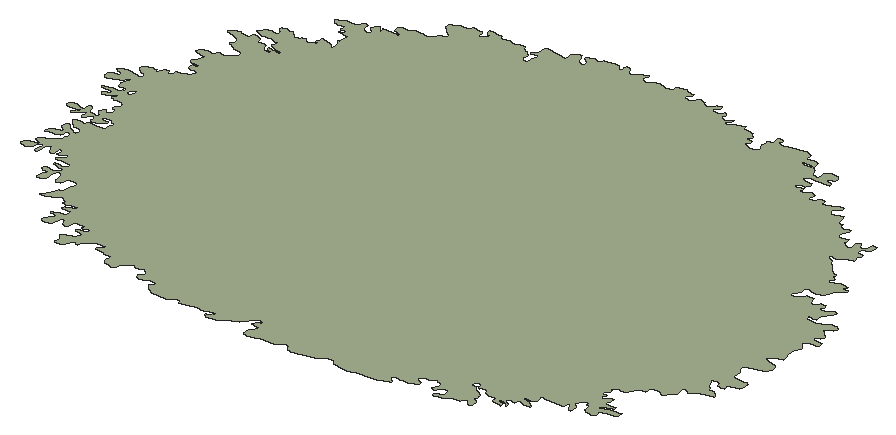
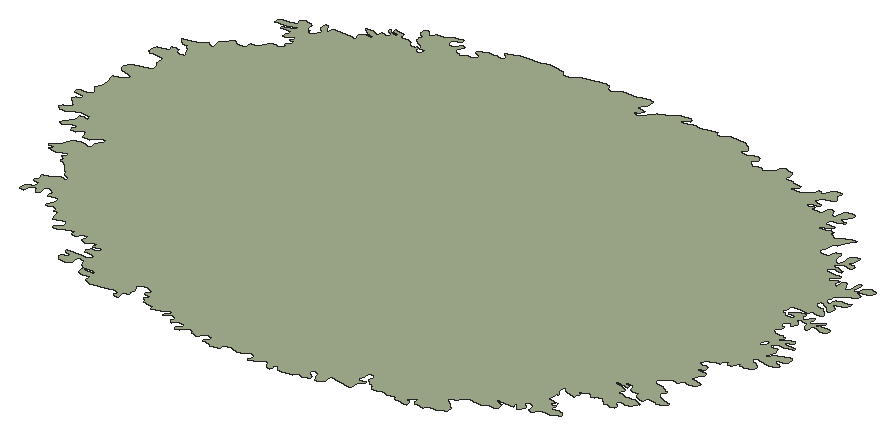
# SketchUp Ruby script. Lengths in inches.
U = 1.inch
M = Sketchup.active_model
def pt(a) = Geom::Point3d.new(a.map { |v| v * U })
def face(e, loops, mat)
  f = e.add_face(loops[0].map { |a| pt(a) })
  loops[1..].each { |l| e.add_face(l.map { |a| pt(a) }).erase! }
  f.material = f.back_material = mat if mat
  f
end
# faces: each face lists its corners as indices into pts; further lists are holes
def faces(e, pts, list, mat = nil) = list.each { |f| face(e, (f[0].is_a?(Array) ? f : [f]).map { |l| l.map { |i| pts[i] } }, mat) }
# xy, xz, yz: faces in a plane at the given z, y or x. An outline is a flat list of corners, or four numbers for a rectangle; further outlines are holes
def ring(l) = l.size == 4 ? [[l[0], l[1]], [l[2], l[1]], [l[2], l[3]], [l[0], l[3]]] : l.each_slice(2).to_a
def flat(e, list, mat, &to3) = list.each { |f| face(e, (f[0].is_a?(Array) ? f : [f]).map { |l| ring(l).map { |u, v| to3.(u, v) } }, mat) }
def xy(e, z, list, mat = nil) = flat(e, list, mat) { |x, y| [x, y, z] }
def xz(e, y, list, mat = nil) = flat(e, list, mat) { |x, z| [x, y, z] }
def yz(e, x, list, mat = nil) = flat(e, list, mat) { |y, z| [x, y, z] }
def lines(e, pts, list) = list.each { |a, b| e.add_line(pt(pts[a]), pt(pts[b])) }
# prism: a flat outline (further loops are holes) pulled along v
def prism(e, loops, v, mat = nil)
  f = face(e, loops, mat); d = Geom::Vector3d.new(v.map { |x| x * U })
  f.pushpull(f.normal.samedirection?(d) ? d.length : -d.length)
end
def box(e, o, s, mat = nil) = prism(e, [[o, [o[0] + s[0], o[1], o[2]], [o[0] + s[0], o[1] + s[1], o[2]], [o[0], o[1] + s[1], o[2]]]], [0, 0, s[2]], mat)
def at(x, y, z, deg = 0) = Geom::Transformation.translation(pt([x, y, z])) * Geom::Transformation.rotation(ORIGIN, Z_AXIS, deg.degrees)
def axes(o, x, y, z) = Geom::Transformation.new([*x, 0, *y, 0, *z, 0, *pt(o).to_a, 1])
def part(name) = M.definitions.add(name)
# library, detail: a bought-in or finely detailed component or shape, given as its bounding box
def library(name, o, s) = part(name).tap { |d| box(d.entities, o, s) }
def detail(e, o, s) = box(e.add_group.entities, o, s)
def put(e, d, t, mat = nil) = e.add_instance(d, t).tap { |i| i.material = mat if mat }
def group(e, t, mat = nil) = e.add_group.tap { |g| g.transformation = t; g.material = mat if mat }.entities
root = M.entities
M.materials.add("Boxwoodplan").color = [166, 177, 144]
xy(root,9.058,[[[143.917,67.129,143.806,67.133,143.711,67.159,143.655,67.215,143.653,67.317,143.679,67.382,143.743,67.445,143.792,67.509,143.85,67.606,143.664,67.635,143.574,67.644,143.594,67.732,143.68,67.79,143.711,67.8,143.706,67.846,143.617,67.877,143.501,67.837,143.404,67.706,143.261,67.551,143.1,67.464,142.995,67.441,142.934,67.416,142.918,67.373,142.774,67.281,142.58,67.251,142.491,67.26,142.411,67.306,142.411,67.328,142.456,67.359,142.547,67.437,142.615,67.483,142.526,67.498,142.413,67.48,142.293,67.436,142.197,67.445,142.1,67.454,142.003,67.447,141.876,67.403,141.676,67.356,141.587,67.349,141.549,67.443,141.541,67.465,141.474,67.473,141.385,67.454,141.216,67.336,141.016,67.328,140.786,67.353,140.619,67.446,140.478,67.61,140.661,67.702,140.561,67.756,140.425,67.772,140.299,67.749,140.227,67.697,140.146,67.672,140.03,67.738,139.988,67.806,140.076,67.847,140.102,67.907,140.107,67.957,140.066,68.009,139.994,68.085,139.908,68.117,139.821,68.064,139.755,68.038,139.699,68.08,139.682,68.103,139.658,68.121,139.629,68.111,139.549,68.058,139.478,68.01,139.402,67.923,139.39,67.79,139.319,67.749,139.269,67.723,139.209,67.725,139.11,67.746,139.023,67.793,138.979,67.861,138.971,67.951,138.98,68.018,138.993,68.04,138.974,68.08,138.76,68.1,138.828,68.135,138.802,68.136,138.709,68.13,138.539,68.146,138.462,68.173,138.445,68.206,138.46,68.224,138.585,68.314,138.583,68.371,138.498,68.393,138.339,68.39,138.208,68.319,138.111,68.233,138.036,68.199,137.989,68.172,137.988,68.154,138.024,68.101,138.008,68.046,137.938,68.081,137.874,68.121,137.813,68.072,137.791,68.017,137.759,67.904,137.712,67.855,137.639,67.822,137.548,67.816,137.478,67.841,137.459,67.874,137.466,67.892,137.487,67.932,137.509,67.991,137.478,68.048,137.377,68.149,137.491,68.229,137.552,68.269,137.632,68.285,137.699,68.315,137.754,68.37,137.839,68.476,137.767,68.503,137.6875,68.511,137.555,68.53,137.517,68.565,137.524,68.584,137.599,68.62,137.761,68.657,137.803,68.709,137.798,68.748,137.772,68.764,137.622,68.711,137.576,68.732,137.577,68.752,137.6,68.814,137.439,68.825,137.358,68.833,137.304,68.826,137.297,68.806,137.281,68.71,137.266,68.642,137.224,68.591,137.177,68.578,137.158,68.594,137.099,68.639,137.054,68.757,137.015,68.783,136.988,68.784,136.934,68.777,136.927,68.757,136.925,68.641,136.871,68.523,136.81,68.449,136.73,68.419,136.651,68.422,136.605,68.448,136.572,68.506,136.572,68.564,136.626,68.677,136.74,68.784,136.76,68.803,136.747,68.823,136.72,68.829,136.64,68.847,136.559,68.86,136.532,68.875,136.539,68.895,136.559,68.914,136.708,68.982,136.87,69.005,136.912,69.108,136.885,69.169,136.838,69.191,136.811,69.187,136.648,69.168,136.607,69.2,136.614,69.22,136.641,69.279,136.799,69.334,136.971,69.403,137.019,69.442,137.006,69.463,136.909,69.436,136.738,69.417,136.594,69.372,136.505,69.386,136.478,69.392,136.484,69.412,136.505,69.426,136.56,69.47,136.532,69.507,136.505,69.503,136.422,69.511,136.367,69.56,136.353,69.601,136.326,69.597,136.243,69.575,136.086,69.489,135.937,69.413,135.863,69.38,135.808,69.392,135.821,69.412,135.84,69.452,135.867,69.469,135.891,69.55,135.941,69.65,135.973,69.759,136.024,69.812,136.097,69.852,136.141,69.972,136.163,70.112,136.183,70.227,136.179,70.285,136.134,70.321,136.053,70.335,135.967,70.335,135.893,70.31,135.883,70.245,135.884,70.184,135.851,70.124,135.763,70.087,135.706,70.096,135.668,70.155,135.657,70.216,135.631,70.337,135.626,70.4,135.585,70.453,135.558,70.475,135.52,70.491,135.461,70.479,135.427,70.46,135.425,70.428,135.417,70.366,135.42,70.229,135.445,70.167,135.437,70.103,135.386,70.038,135.338,70.01,135.3,69.998,135.262,70.003,135.22,70.011,135.202,70.039,135.198,70.166,135.219,70.223,135.264,70.276,135.28,70.306,135.272,70.334,135.215,70.34,135.133,70.346,135.096,70.362,135.073,70.39,135.07,70.453,135.085,70.483,135.12,70.499,135.292,70.472,135.371,70.497,135.42,70.526,135.481,70.573,135.494,70.636,135.471,70.662,135.427,70.664,135.35,70.67,135.258,70.681,135.157,70.717,135.138,70.746,135.144,70.76,135.163,70.763,135.223,70.775,135.398,70.761,135.488,70.787,135.5,70.844,135.474,70.907,135.402,70.946,135.323,70.953,135.21,70.946,135.11,70.921,135.027,70.939,135.023,70.968,135.043,70.997,135.09,71.054,135.156,71.11,135.209,71.19,135.201,71.224,135.156,71.241,135.091,71.24,134.973,71.14,134.933,71.141,134.899,71.161,134.921,71.22,134.937,71.287,134.894,71.35,134.854,71.366,134.834,71.367,134.828,71.352,134.832,71.306,134.829,71.164,134.788,71.102,134.749,71.108,134.714,71.131,134.616,71.262,134.592,71.327,134.567,71.355,134.552,71.344,134.496,71.293,134.461,71.234,134.481,71.103,134.486,71.037,134.466,70.971,134.416,70.962,134.382,70.978,134.372,71.023,134.392,71.155,134.401,71.233,134.401,71.27,134.386,71.282,134.371,71.272,134.292,71.237,134.252,71.183,134.243,71.12,134.204,71.077,134.067,70.987,134.027,70.977,133.983,70.986,133.903,71.026,133.883,71.056,133.887,71.089,133.92,71.151,134.017,71.237,134.107,71.263,134.197,71.263,134.292,71.267,134.231,71.318,134.08,71.404,134.063,71.466,134.116,71.503,134.208,71.573,134.327,71.635,134.445,71.709,134.481,71.723,134.507,71.746,134.533,71.789,134.536,71.882,134.569,72.003,134.57,72.065,134.549,72.086,134.527,72.095,134.464,72.109,134.431,72.104,134.427,72.088,134.439,71.996,134.397,71.934,134.349,71.899,134.272,71.871,134.201,71.858,134.04,71.833,134.005,71.839,133.992,71.853,133.992,71.86,134.001,71.901,134.018,71.947,134.06,71.995,134.129,72.042,134.188,72.063,134.246,72.065,134.285,72.068,134.305,72.075,134.328,72.096,134.323,72.121,134.269,72.151,134.201,72.207,134.169,72.264,134.165,72.331,134.178,72.382,134.23,72.426,134.256,72.432,134.267,72.425,134.287,72.411,134.33,72.35,134.379,72.304,134.507,72.226,134.581,72.192,134.616,72.177,134.636,72.184,134.66,72.206,134.667,72.222,134.678,72.263,134.663,72.32,134.62,72.366,134.588,72.389,134.554,72.401,134.494,72.401,134.42,72.404,134.377,72.446,134.291,72.519,134.232,72.569,134.193,72.617,134.194,72.646,134.218,72.671,134.274,72.698,134.309,72.703,134.35,72.7,134.41,72.679,134.472,72.677,134.508,72.684,134.542,72.726,134.591,72.757,134.65,72.764,134.721,72.764,134.875,72.771,135.015,72.792,135.048,72.808,135.049,72.826,135.043,72.868,135.031,72.913,135.042,72.957,135.072,73.06,135.059,73.083,135.036,73.097,134.979,73.126,134.926,73.164,134.853,73.192,134.78,73.195,134.73,73.184,134.709,73.17,134.684,73.119,134.689,73.098,134.7,73.093,134.724,73.088,134.875,73.076,134.901,73.071,134.906,73.0625,134.897,73.046,134.857,73.007,134.812,72.964,134.747,72.928,134.685,72.884,134.613,72.849,134.576,72.852,134.556,72.863,134.531,72.9,134.524,72.995,134.507,73.02,134.525,73.034,134.531,73.077,134.525,73.088,134.514,73.088,134.499,73.087,134.473,73.083,134.441,73.076,134.423,73.065,134.342,72.97,134.31,72.915,134.279,72.892,134.256,72.895,134.23,72.916,134.221,72.932,134.215,72.973,134.244,73.057,134.249,73.102,134.24,73.13,134.22,73.137,134.182,73.128,134.162,73.114,134.116,73.064,133.994,72.957,133.958,72.932,133.932,72.927,133.895,72.935,133.883,72.951,133.974,73.057,134.037,73.102,134.051,73.129,134.05,73.145,134.041,73.152,134.03,73.148,134.015,73.143,133.984,73.131,133.9,73.108,133.733,73.089,133.66,73.096,133.612,73.121,133.59,73.149,133.589,73.165,133.606,73.217,133.654,73.264,133.714,73.281,133.785,73.284,133.859,73.266,133.987,73.223,134.073,73.197,134.084,73.201,134.084,73.22,134.075,73.239,134.05,73.287,134.049,73.342,134.056,73.407,134.068,73.437,134.085,73.45,134.134,73.413,134.173,73.363,134.2,73.317,134.21,73.255,134.222,73.204,134.237,73.176,134.26,73.175,134.395,73.157,134.468,73.144,134.503,73.14,134.521,73.154,134.536,73.202,134.481,73.244,134.422,73.309,134.405,73.335,134.405,73.352,134.439,73.46,134.469,73.483,134.496,73.489,134.511,73.477,134.52,73.459,134.549,73.414,134.56,73.39,134.572,73.391,134.593,73.404,134.673,73.482,134.69,73.528,134.691,73.579,134.677,73.611,134.656,73.623,134.593,73.646,134.553,73.666,134.545,73.687,134.561,73.736,134.617,73.773,134.651,73.795,134.664,73.816,134.672,73.869,134.67,73.916,134.575,73.992,134.431,74.014,134.369,74.031,134.334,74.013,134.306,74.014,134.237,74.031,134.218,74.058,134.227,74.082,134.353,74.185,134.347,74.217,134.325,74.233,134.28,74.225,134.251,74.216,134.125,74.154,134.085,74.107,134.036,74.063,133.967,74.049,133.939,74.05,133.892,74.102,133.92,74.126,133.9375,74.165,133.969,74.188,134.063,74.22,134.108,74.25,134.097,74.281,134.084,74.283,134.074,74.276,134.048,74.27,134.009,74.273,133.874,74.284,133.727,74.3125,133.703,74.327,133.709,74.347,133.734,74.375,133.947,74.435,134.01,74.434,134.071,74.419,134.131,74.391,134.158,74.393,134.164,74.403,134.213,74.48,134.237,74.495,134.243,74.515,134.243,74.583,134.232,74.593,134.219,74.591,134.161,74.591,134.104,74.585,134.057,74.568,134.033,74.576,134.012,74.596,133.987,74.63,133.967,74.718,133.978,74.806,134.008,74.848,134.014,74.88,134.027,74.923,134.064,74.944,134.06,74.99,134.038,75.026,133.949,75.003,133.931,74.969,133.932,74.95,133.935,74.886,133.855,74.839,133.714,74.745,133.558,74.7,133.474,74.725,133.432,74.778,133.423,74.904,133.551,74.99,133.634,75.003,133.677,75.027,133.701,75.061,133.7,75.081,133.614,75.112,133.541,75.138,133.479,75.194,133.514,75.249,133.59,75.278,133.686,75.312,133.751,75.311,133.93,75.267,134.022,75.246,134.107,75.25,134.158,75.269,134.164,75.289,134.148,75.355,134.087,75.407,134.042,75.415,133.93,75.485,133.883,75.527,133.869,75.564,133.862,75.617,133.862,75.644,133.875,75.659,133.917,75.695,133.968,75.709,134.082,75.741,134.113,75.751,134.153,75.75,134.203,75.746,134.216,75.733,134.231,75.703,134.245,75.689,134.255,75.689,134.283,75.692,134.299,75.704,134.32,75.754,134.348,75.787,134.364,75.81,134.367,75.835,134.383,75.86,134.403,75.872,134.451,75.884,134.49,75.877,134.511,75.833,134.515,75.781,134.532,75.755,134.553,75.754,134.595,75.796,134.62,75.838,134.634,75.942,134.65,75.968,134.682,75.975,134.714,75.974,134.733,75.963,134.754,75.94,134.786,75.94,134.839,75.961,134.883,76.007,134.897,76.032,134.886,76.046,134.946,76.043,134.975,76.046,134.991,76.066,134.996,76.114,135.03,76.155,135.064,76.2,135.01,76.243,134.943,76.272,134.906,76.271,134.873,76.261,134.831,76.249,134.789,76.255,134.767,76.271,134.746,76.295,134.723,76.397,134.736,76.423,134.741,76.439,134.751,76.443,134.856,76.463,134.902,76.472,134.92,76.483,134.91,76.486,134.824,76.514,134.758,76.526,134.73,76.519,134.695,76.52,134.659,76.52,134.623,76.532,134.585,76.582,134.567,76.611,134.567,76.642,134.582,76.663,134.611,76.678,134.642,76.697,134.65,76.725,134.68,76.782,134.707,76.836,134.713,76.89,134.706,76.917,134.666,76.928,134.588,76.954,134.415,77.001,134.379,77.018,134.362,77.042,134.398,77.097,134.442,77.131,134.488,77.159,134.543,77.178,134.595,77.1875,134.648,77.184,134.703,77.16,134.758,77.162,134.785,77.167,134.798,77.187,134.815,77.228,134.852,77.264,134.873,77.282,134.899,77.284,134.968,77.267,135.03,77.256,135.056,77.253,135.08,77.268,135.167,77.336,135.254,77.401,135.308,77.498,135.304,77.542,135.263,77.579,135.146,77.617,135.02,77.647,134.934,77.719,134.876,77.755,134.807,77.776,134.78,77.788,134.766,77.808,134.788,77.855,134.836,77.896,134.834,77.981,134.784,78.06,134.654,78.116,134.366,78.212,134.345,78.246,134.417,78.31,134.538,78.362,134.643,78.367,134.7,78.353,134.744,78.327,134.793,78.317,134.846,78.326,134.907,78.337,134.936,78.368,134.951,78.448,134.968,78.483,135.022,78.482,135.079,78.471,135.127,78.451,135.194,78.392,135.218,78.358,135.232,78.318,135.233,78.249,135.239,78.245,135.248,78.249,135.275,78.262,135.326,78.268,135.415,78.271,135.495,78.235,135.529,78.17,135.554,78.092,135.624,78.047,135.664,78.035,135.682,78.034,135.709,78.043,135.804,78.05,135.821,78.055,135.801,78.071,135.738,78.095,135.686,78.099,135.648,78.118,135.629,78.152,135.626,78.164,135.629,78.184,135.644,78.191,135.679,78.192,135.721,78.185,135.827,78.156,135.942,78.152,135.994,78.159,136.012,78.162,136.038,78.173,135.994,78.203,135.953,78.213,135.867,78.228,135.809,78.242,135.768,78.244,135.746,78.248,135.721,78.263,135.669,78.289,135.622,78.315,135.6,78.348,135.61,78.404,135.639,78.442,135.68,78.471,135.64,78.502,135.585,78.517,135.542,78.52,135.487,78.528,135.456,78.555,135.438,78.591,135.424,78.6,135.395,78.599,135.279,78.571,135.227,78.557,135.178,78.559,135.13,78.562,135.081,78.578,135.033,78.595,134.993,78.602,134.907,78.65,134.932,78.662,134.934,78.669,134.945,78.709,134.961,78.745,134.987,78.782,135.018,78.814,135.062,78.839,135.115,78.862,135.16,78.873,135.266,78.867,135.343,78.862,135.376,78.858,135.387,78.857,135.387,78.87,135.379,78.912,135.358,78.956,135.322,78.995,135.279,79.026,135.246,79.073,135.248,79.096,135.259,79.117,135.306,79.147,135.358,79.17,135.385,79.169,135.411,79.163,135.465,79.148,135.533,79.142,135.58,79.127,135.604,79.114,135.622,79.095,135.666,79.055,135.705,79.02,135.75,78.989,135.806,78.976,135.86,78.981,135.905,79.01,135.937,79.046,135.986,79.084,136.012,79.083,136.034,79.069,136.075,79.027,136.122,78.994,136.25,79.019,136.324,79.037,136.365,79.065,136.371,79.085,136.35,79.102,136.299,79.124,136.289,79.147,136.297,79.169,136.313,79.214,136.32,79.273,136.324,79.299,136.347,79.315,136.374,79.316,136.404,79.308,136.446,79.288,136.58,79.248,136.641,79.226,136.68,79.193,136.707,79.153,136.722,79.13,136.729,79.123,136.738,79.126,136.746,79.131,136.779,79.176,136.785,79.212,136.775,79.315,136.753,79.362,136.729,79.397,136.694,79.436,136.684,79.466,136.695,79.477,136.706,79.475,136.728,79.476,136.727,79.484,136.732,79.508,136.725,79.549,136.71,79.705,136.712,79.782,136.597,79.802,136.5,79.804,136.4375,79.8125,136.42,79.819,136.406,79.83,136.419,79.839,136.532,79.882,136.566,79.911,136.565,79.924,136.542,79.948,136.506,79.952,136.453,79.94,136.405,79.918,136.388,79.919,136.373,79.945,136.399,80.028,136.402,80.069,136.401,80.082,136.377,80.103,136.288,80.085,136.175,80.088,136.066,80.105,136.005,80.185,136.003,80.213,136.041,80.25,136.137,80.303,136.186,80.33,136.24,80.335,136.365,80.332,136.456,80.337,136.516,80.346,136.556,80.384,136.596,80.418,136.604,80.461,136.63,80.5,136.686,80.513,136.723,80.509,136.766,80.475,136.777,80.389,136.784,80.3,136.808,80.257,136.863,80.231,136.955,80.212,137.01,80.234,137.028,80.276,137.005,80.319,136.958,80.355,136.902,80.442,136.938,80.521,137.012,80.603,137.031,80.606,137.055,80.576,137.074,80.528,137.148,80.447,137.176,80.421,137.167,80.475,137.149,80.57,137.205,80.587,137.266,80.582,137.393,80.578,137.506,80.575,137.628,80.557,137.646,80.557,137.634,80.587,137.583,80.629,137.453,80.681,137.415,80.689,137.392,80.735,137.394,80.826,137.429,80.871,137.478,80.896,137.594,80.901,137.691,80.91,137.786,80.977,137.912,80.982,138.028,80.971,138.124,80.953,138.245,80.946,138.288,80.991,138.301,81.038,138.344,81.133,138.433,81.187,138.553,81.244,138.565,81.26,138.548,81.294,138.507,81.332,138.4,81.413,138.332,81.487,138.274,81.528,138.217,81.57,138.248,81.577,138.247,81.591,138.242,81.612,138.231,81.679,138.234,81.709,138.269,81.744,138.352,81.785,138.435,81.821,138.473,81.827,138.529,81.826,138.616,81.816,138.639,81.808,138.663,81.81,138.695,81.843,138.747,81.918,138.783,81.932,138.84,81.936,138.942,81.93,139.038,81.898,139.07,81.877,139.099,81.835,139.1,81.765,139.103,81.736,139.108,81.715,139.131,81.704,139.184,81.715,139.229,81.745,139.291,81.798,139.316,81.822,139.337,81.834,139.35,81.85,139.265,81.897,139.227,81.913,139.184,81.956,139.159,82.036,139.16,82.067,139.218,82.083,139.41,82.055,139.507,82.039,139.542,82.026,139.542,81.98,139.552,81.952,139.612,81.948,139.716,81.962,139.818,81.975,139.86,81.971,139.907,81.957,139.934,81.934,139.959,81.933,139.984,81.943,140.128,81.972,140.169,81.981,140.221,81.987,140.257,81.984,140.302,81.957,140.332,81.886,140.358,81.863,140.403,81.844,140.443,81.833,140.483,81.808,140.535,81.753,140.589,81.696,140.576,81.619,140.569,81.545,140.583,81.515,140.614,81.485,140.641,81.461,140.688,81.453,140.724,81.45,140.769,81.481,140.782,81.512,140.783,81.553,140.771,81.628,140.808,81.787,140.797,81.817,140.779,81.829,140.755,81.833,140.716,81.834,140.664,81.828,140.628,81.826,140.581,81.835,140.556,81.858,140.563,81.88,140.591,81.896,140.63,81.91,140.675,81.937,140.7,82.013,140.704,82.178,140.704,82.21,140.727,82.228,140.753,82.233,140.852,82.222,141.051,82.201,141.142,82.19,141.231,82.169,141.318,82.153,141.369,82.147,141.364,82.355,141.432,82.427,141.517,82.486,141.571,82.477,141.599,82.441,141.647,82.37,141.67,82.297,141.678,82.26,141.676,82.241,141.703,82.206,141.808,82.173,141.86,82.173,141.899,82.204,141.902,82.279,141.799,82.36,141.721,82.419,141.733,82.453,141.777,82.49,141.871,82.541,141.921,82.55,142.002,82.538,142.106,82.537,142.129,82.615,142.339,82.643,142.439,82.661,142.547,82.647,142.626,82.578,142.659,82.543,142.686,82.541,142.726,82.568,142.724,82.643,142.715,82.685,142.728,82.72,142.778,82.729,142.833,82.715,142.904,82.621,142.925,82.548,142.958,82.513,143.007,82.498,143.058,82.503,143.104,82.53,143.192,82.613,143.273,82.668,143.375,82.715,143.423,82.7,143.437,82.663,143.385,82.592,143.359,82.557,143.367,82.515,143.456,82.457,143.556,82.443,143.606,82.452,143.656,82.498,143.734,82.566,143.849,82.581,143.964,82.553,143.995,82.523,144.072,82.492,144.172,82.511,144.254,82.565,144.254,82.678,144.311,82.721,144.424,82.745,144.529,82.74,144.61,82.681,144.756,82.66,144.81,82.651,144.816,82.614,144.742,82.546,144.709,82.473,144.721,82.437,144.793,82.396,144.895,82.401,144.948,82.433,144.968,82.472,144.988,82.544,145.037,82.567,145.061,82.579,145.112,82.579,145.215,82.541,145.258,82.47,145.344,82.417,145.474,82.447,145.509,82.478,145.515,82.52,145.555,82.603,145.662,82.622,145.692,82.592,145.698,82.55,145.645,82.466,145.597,82.448,145.57,82.413,145.63,82.349,145.761,82.337,145.852,82.373,145.919,82.444,145.944,82.45,145.953,82.433,145.971,82.392,145.995,82.357,145.984,82.301,145.964,82.257,145.982,82.222,146.071,82.179,146.179,82.184,146.234,82.203,146.285,82.258,146.302,82.273,146.304,82.255,146.291,82.212,146.218,82.132,146.184,82.102,146.195,82.066,146.242,82.047,146.3,82.048,146.396,82.088,146.478,82.146,146.698,82.225,146.72,82.153,146.743,82.123,146.794,82.118,146.91,82.11,147.034,82.084,147.049,82.013,147.072,81.983,147.118,81.964,147.141,81.93,147.127,81.892,147.1,81.795,147.217,81.773,147.263,81.755,147.273,81.72,147.199,81.65,147.185,81.613,147.201,81.579,147.277,81.527,147.38,81.5,147.481,81.496,147.593,81.563,147.635,81.639,147.577,81.71,147.544,81.779,147.564,81.885,147.573,81.922,147.544,81.956,147.54,81.992,147.582,82.018,147.683,82.022,147.672,82.122,147.63,82.274,147.68,82.287,147.745,82.275,147.798,82.256,147.829,82.199,147.779,82.131,147.783,82.095,147.829,82.076,147.937,82.076,148.067,82.111,148.574,82.178,148.62,82.168,148.666,82.145,148.712,82.121,148.746,82.097,148.777,82.027,148.76,81.935,148.964,81.949,149.029,81.943,149.114,81.911,149.151,81.805,149.136,81.757,149.12,81.724,149.079,81.717,148.909,81.749,148.845,81.755,148.802,81.755,148.782,81.749,148.779,81.733,148.807,81.685,148.848,81.666,148.895,81.666,149.068,81.681,149.137,81.683,149.221,81.648,149.258,81.609,149.289,81.546,149.357,81.437,149.436,81.398,149.521,81.394,149.552,81.435,149.546,81.518,149.528,81.571,149.535,81.637,149.576,81.687,149.677,81.719,149.786,81.732,149.875,81.701,149.923,81.659,149.957,81.597,149.958,81.551,149.896,81.495,149.83,81.482,149.789,81.471,149.757,81.437,149.761,81.407,149.81,81.389,149.908,81.363,149.979,81.339,149.999,81.306,149.987,81.275,149.933,81.247,149.846,81.24,149.684,81.233,149.597,81.222,149.508,81.256,149.444,81.269,149.362,81.251,149.306,81.208,149.304,81.143,149.362,81.103,149.449,81.081,149.535,81.066,149.582,81.066,149.616,81.046,149.637,81.003,149.62,80.938,149.585,80.89,149.557,80.866,149.512,80.854,149.37,80.834,149.35,80.829,149.341,80.784,149.345,80.751,149.39,80.732,149.457,80.731,149.498,80.731,149.548,80.746,149.611,80.778,149.625,80.712,149.596,80.665,149.589,80.635,149.628,80.617,149.689,80.622,149.771,80.67,149.827,80.711,149.855,80.736,149.893,80.721,149.957,80.704,150.026,80.651,150.022,80.603,149.979,80.537,149.946,80.472,149.964,80.448,150.011,80.445,150.087,80.456,150.169,80.495,150.208,80.554,150.28,80.597,150.34,80.609,150.377,80.601,150.395,80.577,150.398,80.548,150.381,80.521,150.353,80.497,150.355,80.483,150.376,80.481,150.548,80.499,150.629,80.51,150.696,80.552,150.738,80.589,150.817,80.614,150.914,80.619,150.937,80.595,150.94,80.566,150.78,80.349,150.795,80.304,150.852,80.251,150.935,80.237,151.024,80.255,151.092,80.283,151.177,80.305,151.242,80.213,151.278,79.999,151.28,79.985,151.316,79.974,151.4,79.996,151.411,79.918,151.435,79.871,151.511,79.861,151.648,79.896,151.716,79.893,151.731,79.839,151.663,79.619,151.652,79.567,151.675,79.514,151.741,79.486,151.809,79.496,151.945,79.523,151.965,79.419,151.96,79.316,152.082,79.247,152.215,79.216,152.245,79.318,152.235,79.421,152.212,79.474,152.24,79.525,152.309,79.535,152.348,79.482,152.37,79.429,152.418,79.395,152.495,79.418,152.549,79.467,152.573,79.583,152.577,79.636,152.638,79.659,152.695,79.631,152.725,79.577,152.7,79.455,152.585,79.375,152.532,79.339,152.511,79.282,152.491,79.231,152.514,79.186,152.646,79.161,152.702,79.134,152.707,79.083,152.634,78.997,152.669,78.895,152.698,78.844,152.686,78.794,152.552,78.768,152.451,78.729,152.347,78.658,152.296,78.623,152.23,78.626,152.166,78.659,152.134,78.667,152.108,78.643,152.152,78.549,152.271,78.483,152.318,78.445,152.315,78.396,152.4,78.32,152.566,78.132,152.698,78.05,152.761,78.035,152.798,77.992,152.783,77.898,152.899,77.834,152.836,77.749,152.816,77.697,152.814,77.673,152.845,77.661,152.982,77.679,153.117,77.755,153.247,77.768,153.372,77.734,153.375,77.687,153.309,77.66,153.283,77.644,153.297,77.62,153.375,77.599,153.447,77.596,153.479,77.595,153.492,77.571,153.404,77.482,153.238,77.322,153.214,77.232,153.21,77.187,153.182,77.142,153.089,77.067,152.961,77.038,152.836,77.043,152.727,77.082,152.658,77.076,152.631,77.004,152.658,76.894,152.629,76.787,152.511,76.72,152.539,76.62,152.677,76.642,152.849,76.833,153.076,76.815,153.152,76.605,153.197,76.595,153.279,76.618,153.366,76.723,153.504,76.735,153.542,76.635,153.492,76.574,153.477,76.539,153.554,76.501,153.693,76.531,153.8125,76.598,153.859,76.614,153.949,76.592,153.927,76.477,153.816,76.384,153.751,76.289,153.759,76.113,153.745,76.078,153.652,76.056,153.52,76.087,153.545,75.981,153.676,75.941,153.822,75.936,153.971,75.965,154.208,76.087,154.344,76.099,154.436,76.008,154.403,75.905,154.263,75.849,154.216,75.825,154.1875,75.766,154.291,75.675,154.442,75.515,154.409,75.414,154.293,75.359,154.257,75.335,154.295,75.274,154.439,75.269,154.569,75.247,154.581,75.145,154.508,75.089,154.375,75.078,154.25,75.041,154.207,74.942,154.375,74.761,154.268,74.568,154.271,74.388,154.325,74.176,154.369,74.078,154.237,74.051,154.114,74.008,154.02,73.931,153.993,73.869,154.104,73.801,154.356,73.744,154.433,73.662,154.454,73.559,154.412,73.467,154.297,73.394,153.836,73.234,153.838,73.141,153.882,73.048,153.936,72.954,153.9375,72.863,153.932,72.803,153.929,72.773,153.955,72.719,154.076,72.676,154.201,72.672,154.327,72.682,154.369,72.68,154.427,72.633,154.438,72.453,154.411,72.395,154.302,72.347,154.175,72.33,154.134,72.331,154.088,72.281,154.13,72.191,154.117,72.163,154.032,72.144,153.991,72.145,153.921,72.17,153.889,72.26,153.819,72.292,153.696,72.297,153.654,72.291,153.638,72.233,153.714,72.156,153.801,71.992,153.829,71.969,153.855,71.918,153.873,71.888,153.954,71.877,154.034,71.86,154.119,71.792,154.182,71.71,154.179,71.681,154.095,71.656,153.846,71.616,153.651,71.488,153.578,71.469,153.483,71.544,153.443,71.553,153.379,71.52,153.382,71.435,153.438,71.27,153.396,71.264,153.363,71.219,153.314,71.18,153.26,71.066,153.221,71.019,153.187,71,153.151,71.013,153.029,71.1,152.966,71.115,152.923,71.116,152.878,71.098,152.815,71.063,152.785,70.991,152.795,70.938,152.777,70.874,152.615,70.852,152.563,70.81,152.531,70.759,152.484,70.718,152.472,70.655,152.441,70.609,152.407,70.583,152.37,70.573,152.301,70.564,152.203,70.575,152.143,70.55,152.081,70.502,152.051,70.457,152.126,70.419,152.153,70.376,152.117,70.32,152.062,70.284,152.041,70.225,152.04,70.209,152.039,70.194,152.058,70.186,152.13,70.18,152.156,70.182,152.176,70.182,152.18,70.166,152.142,70.097,152.123,70.049,152.12,70.02,152.161,70.018,152.3,70.094,152.369,70.11,152.45,70.107,152.434,70.004,152.416,69.89,152.416,69.843,152.439,69.82,152.479,69.818,152.543,69.845,152.624,69.846,152.683,69.832,152.723,69.827,152.729,69.798,152.689,69.76,152.61,69.73,152.544,69.722,152.461,69.696,152.422,69.658,152.405,69.602,152.409,69.587,152.449,69.586,152.531,69.611,152.689,69.673,152.843,69.703,152.969,69.705,153.021,69.685,152.996,69.611,152.975,69.569,152.914,69.518,152.761,69.492,152.622,69.491,152.561,69.482,152.53,69.427,152.556,69.308,152.541,69.264,152.46,69.243,152.324,69.255,152.266,69.261,152.222,69.314,152.213,69.426,152.213,69.468,152.201,69.496,152.192,69.511,152.172,69.512,152.114,69.525,152.109,69.581,152.111,69.595,152.107,69.61,152.088,69.614,152.008,69.617,151.951,69.591,151.906,69.536,151.869,69.499,151.844,69.44,151.855,69.391,151.911,69.354,151.986,69.254,151.982,69.155,151.973,69.115,151.966,69.088,151.935,69.066,151.915,69.067,151.894,69.098,151.865,69.157,151.8,69.258,151.759,69.298,151.745,69.312,151.734,69.299,151.727,69.271,151.724,69.227,151.705,69.173,151.699,69.16,151.669,69.144,151.586,69.137,151.445,69.139,151.159,69.14,151.101,69.162,151.014,69.173,150.995,69.163,150.989,69.133,151.039,69.074,151.064,68.976,151.058,68.936,151.026,68.896,151.002,68.889,150.942,68.88,150.839,68.88,150.741,68.884,150.693,68.853,150.748,68.829,150.849,68.814,150.957,68.78,151.032,68.726,151.113,68.654,151.095,68.629,151.034,68.614,150.933,68.621,150.896,68.63,150.845,68.65,150.797,68.684,150.747,68.708,150.712,68.63,150.702,68.558,150.662,68.545,150.606,68.558,150.561,68.589,150.548,68.6,150.53,68.608,150.518,68.59,150.484,68.513,150.486,68.485,150.519,68.448,150.611,68.416,150.65,68.383,150.663,68.34,150.661,68.326,150.642,68.323,150.599,68.36,150.519,68.409,150.426,68.427,150.369,68.429,150.357,68.415,150.378,68.39,150.492,68.347,150.529,68.335,150.552,68.292,150.548,68.264,150.547,68.251,150.504,68.249,150.391,68.26,150.286,68.295,150.251,68.325,150.242,68.371,150.241,68.441,150.19,68.461,150.131,68.442,150.031,68.449,149.932,68.467,149.905,68.489,149.88,68.526,149.884,68.568,149.89,68.583,149.852,68.591,149.758,68.616,149.701,68.619,149.666,68.606,149.654,68.577,149.634,68.571,149.607,68.597,149.604,68.612,149.634,68.635,149.65,68.646,149.642,68.671,149.555,68.729,149.518,68.752,149.499,68.756,149.458,68.736,149.418,68.716,149.398,68.71,149.387,68.681,149.41,68.59,149.505,68.587,149.544,68.582,149.574,68.541,149.567,68.513,149.561,68.499,149.569,68.471,149.68,68.434,149.768,68.396,149.829,68.338,149.846,68.3125,149.845,68.299,149.81,68.283,149.79,68.273,149.821,68.251,149.876,68.225,149.888,68.2,149.837,68.168,149.825,68.141,149.85,68.106,149.935,68.062,150.013,67.994,150.012,67.851,149.991,67.825,149.939,67.814,149.885,67.829,149.847,67.874,149.807,67.939,149.789,67.949,149.751,67.944,149.699,67.926,149.677,67.897,149.678,67.854,149.677,67.84,149.644,67.828,149.467,67.819,149.459,67.826,149.411,67.808,149.367,67.777,149.283,67.692,149.231,67.661,149.157,67.651,149.019,67.643,148.965,67.658,148.963,67.698,149.072,67.762,149.172,67.834,149.169,67.937,149.163,67.98,149.163,67.994,149.132,68.015,149.072,68.034,148.998,68.034,148.914,67.95,148.894,67.911,148.837,67.866,148.822,67.857,148.786,67.865,148.749,67.88,148.737,67.907,148.777,67.999,148.837,68.094,148.838,68.135,148.77,68.189,148.659,68.224,148.607,68.246,148.57,68.238,148.545,68.215,148.511,68.171,148.478,68.156,148.436,68.157,148.38,68.166,148.343,68.168,148.305,68.145,148.224,68.05,148.238,68.01,148.312,67.97,148.367,67.938,148.394,67.917,148.403,67.89,148.379,67.851,148.319,67.807,148.217,67.756,148.162,67.735,148.089,67.738,148.034,67.76,147.96,67.769,147.915,67.745,147.878,67.743,147.846,67.76,147.791,67.766,147.718,67.752,147.696,67.717,147.706,67.659,147.803,67.575,147.83,67.536,147.831,67.51,147.831,67.497,147.813,67.492,147.523,67.391,147.248,67.369,147.015,67.373,146.924,67.371,146.802,67.31,146.699,67.275,146.602,67.279,146.564,67.281,146.515,67.299,146.467,67.328,146.406,67.325,146.317,67.334,146.233,67.376,146.173,67.433,146.142,67.478,146.083,67.491,145.984,67.479,145.888,67.438,145.808,67.398,145.709,67.325,145.612,67.269,145.519,67.24,145.278,67.222,145.088,67.186,144.991,67.19,144.926,67.284,144.895,67.351,144.807,67.365,144.716,67.352,144.62,67.28,144.555,67.217,144.465,67.21,144.288,67.233,144.103,67.24,144.025,67.189],[134.425,74.415,134.467,74.419,134.487,74.422,134.513,74.431,134.525,74.474,134.526,74.513,134.533,74.597,134.525,74.631,134.513,74.643,134.513,74.658,134.47,74.635,134.414,74.612,134.394,74.606,134.378,74.59,134.357,74.557,134.347,74.52,134.349,74.476,134.368,74.437,134.387,74.421]]],"Boxwoodplan")
